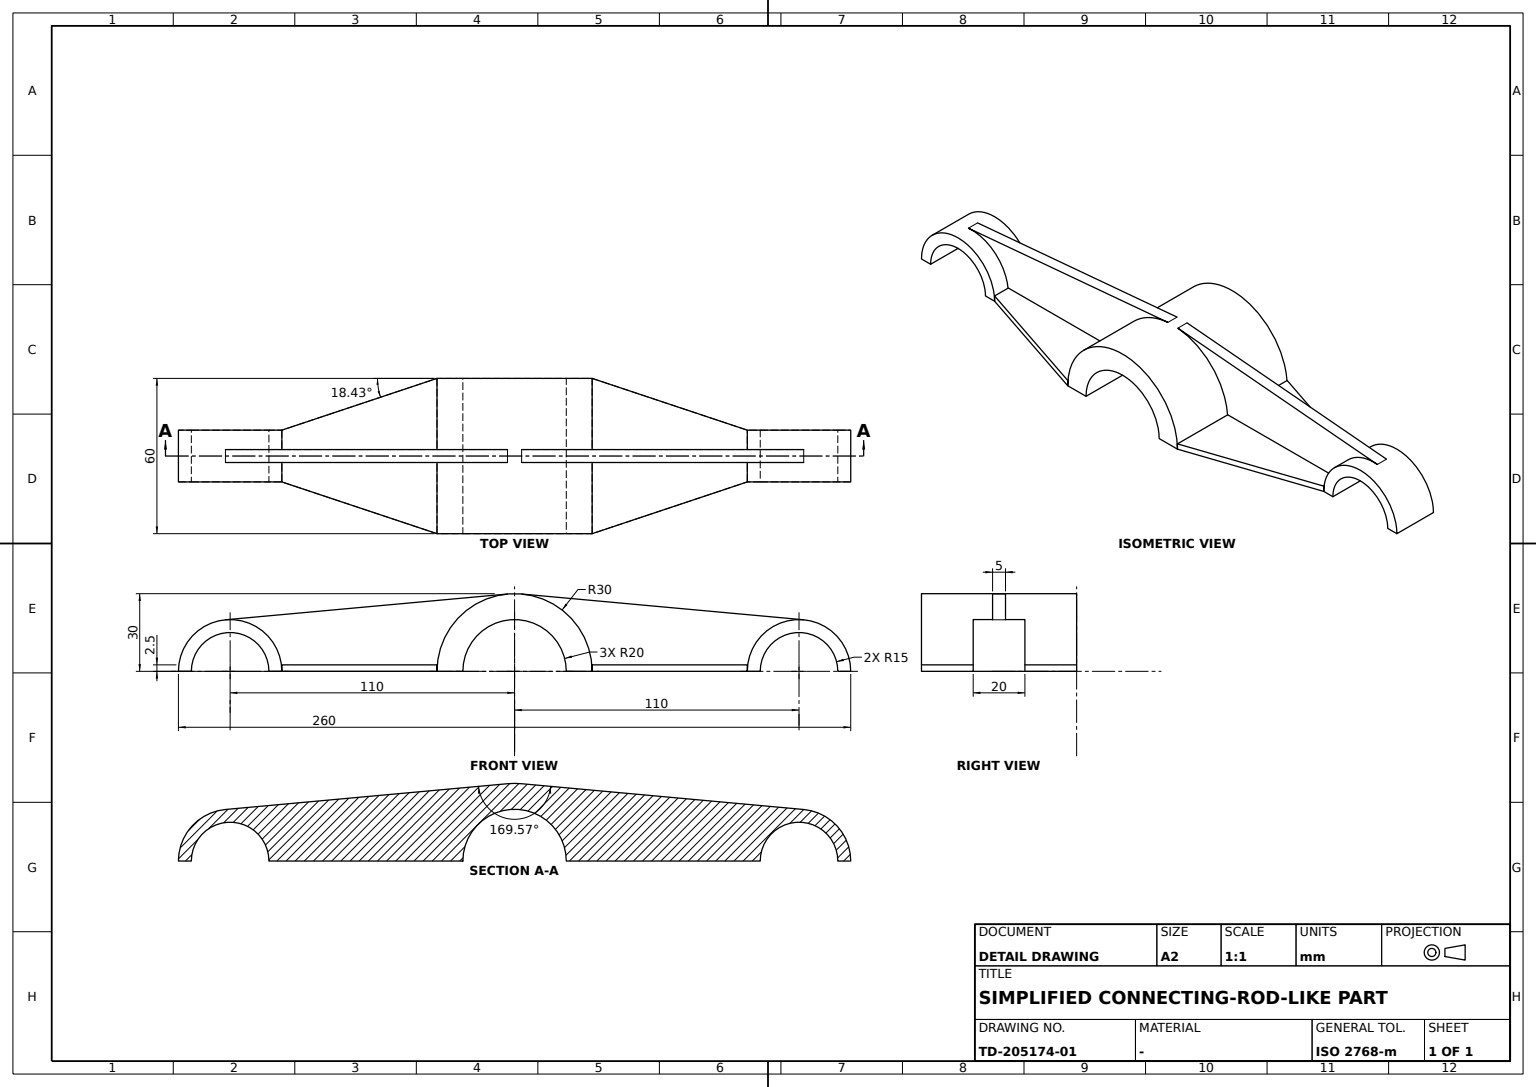
ISO-10303-21;
HEADER;
FILE_DESCRIPTION((''),'2;1');
FILE_NAME('','',(''),(''),'','','');
FILE_SCHEMA(('AUTOMOTIVE_DESIGN'));
ENDSEC;
DATA;
#1=APPLICATION_CONTEXT('');
#2=PRODUCT_CONTEXT('',#1,'mechanical');
#3=PRODUCT('','','',(#2));
#4=PRODUCT_DEFINITION_FORMATION('','',#3);
#5=PRODUCT_DEFINITION_CONTEXT('',#1,'design');
#6=PRODUCT_DEFINITION('','',#4,#5);
#7=PRODUCT_DEFINITION_SHAPE('','',#6);
#8=(LENGTH_UNIT()NAMED_UNIT(*)SI_UNIT(.MILLI.,.METRE.));
#9=(NAMED_UNIT(*)PLANE_ANGLE_UNIT()SI_UNIT($,.RADIAN.));
#10=(NAMED_UNIT(*)SI_UNIT($,.STERADIAN.)SOLID_ANGLE_UNIT());
#11=UNCERTAINTY_MEASURE_WITH_UNIT(LENGTH_MEASURE(0.005),#8,'distance_accuracy_value','');
#12=(GEOMETRIC_REPRESENTATION_CONTEXT(3)GLOBAL_UNCERTAINTY_ASSIGNED_CONTEXT((#11))GLOBAL_UNIT_ASSIGNED_CONTEXT((#8,#9,#10))REPRESENTATION_CONTEXT('',''));
#13=CARTESIAN_POINT('',(20.,-30.,0.));
#14=VERTEX_POINT('',#13);
#15=CARTESIAN_POINT('',(20.,30.,0.));
#16=VERTEX_POINT('',#15);
#17=DIRECTION('',(0.,1.,0.));
#18=VECTOR('',#17,1000.);
#19=LINE('',#13,#18);
#20=EDGE_CURVE('',#14,#16,#19,.T.);
#21=ORIENTED_EDGE('',*,*,#20,.T.);
#22=CARTESIAN_POINT('',(30.,30.,0.));
#23=VERTEX_POINT('',#22);
#24=CARTESIAN_POINT('',(0.,30.,0.));
#25=DIRECTION('',(-1.,0.,0.));
#26=VECTOR('',#25,1000.);
#27=LINE('',#24,#26);
#28=EDGE_CURVE('',#23,#16,#27,.T.);
#29=ORIENTED_EDGE('',*,*,#28,.F.);
#30=CARTESIAN_POINT('',(90.,10.,0.));
#31=VERTEX_POINT('',#30);
#32=DIRECTION('',(0.948683298,-0.316227766,0.));
#33=VECTOR('',#32,1000.);
#34=LINE('',#22,#33);
#35=EDGE_CURVE('',#23,#31,#34,.T.);
#36=ORIENTED_EDGE('',*,*,#35,.T.);
#37=CARTESIAN_POINT('',(95.,10.,0.));
#38=VERTEX_POINT('',#37);
#39=CARTESIAN_POINT('',(30.,10.,0.));
#40=DIRECTION('',(1.,0.,0.));
#41=VECTOR('',#40,1000.);
#42=LINE('',#39,#41);
#43=EDGE_CURVE('',#31,#38,#42,.T.);
#44=ORIENTED_EDGE('',*,*,#43,.T.);
#45=CARTESIAN_POINT('',(95.,-10.,0.));
#46=VERTEX_POINT('',#45);
#47=LINE('',#45,#18);
#48=EDGE_CURVE('',#46,#38,#47,.T.);
#49=ORIENTED_EDGE('',*,*,#48,.F.);
#50=CARTESIAN_POINT('',(90.,-10.,0.));
#51=VERTEX_POINT('',#50);
#52=CARTESIAN_POINT('',(30.,-10.,0.));
#53=LINE('',#52,#41);
#54=EDGE_CURVE('',#51,#46,#53,.T.);
#55=ORIENTED_EDGE('',*,*,#54,.F.);
#56=CARTESIAN_POINT('',(30.,-30.,0.));
#57=VERTEX_POINT('',#56);
#58=DIRECTION('',(0.948683298,0.316227766,0.));
#59=VECTOR('',#58,1000.);
#60=LINE('',#56,#59);
#61=EDGE_CURVE('',#57,#51,#60,.T.);
#62=ORIENTED_EDGE('',*,*,#61,.F.);
#63=CARTESIAN_POINT('',(0.,-30.,0.));
#64=LINE('',#63,#26);
#65=EDGE_CURVE('',#57,#14,#64,.T.);
#66=ORIENTED_EDGE('',*,*,#65,.T.);
#67=EDGE_LOOP('',(#21,#29,#36,#44,#49,#55,#62,#66));
#68=FACE_BOUND('',#67,.T.);
#69=CARTESIAN_POINT('',(30.,0.,0.));
#70=DIRECTION('',(0.,0.,-1.));
#71=AXIS2_PLACEMENT_3D('',#69,#70,#25);
#72=PLANE('',#71);
#73=ADVANCED_FACE('',(#68),#72,.T.);
#74=ORIENTED_EDGE('',*,*,#20,.F.);
#75=CARTESIAN_POINT('',(-20.,-30.,0.));
#76=VERTEX_POINT('',#75);
#77=DIRECTION('',(0.,0.,1.));
#78=AXIS2_PLACEMENT_3D('',#63,#17,#77);
#79=CIRCLE('',#78,20.);
#80=EDGE_CURVE('',#76,#14,#79,.T.);
#81=ORIENTED_EDGE('',*,*,#80,.F.);
#82=CARTESIAN_POINT('',(-20.,30.,0.));
#83=VERTEX_POINT('',#82);
#84=LINE('',#75,#18);
#85=EDGE_CURVE('',#76,#83,#84,.T.);
#86=ORIENTED_EDGE('',*,*,#85,.T.);
#87=AXIS2_PLACEMENT_3D('',#24,#17,#77);
#88=CIRCLE('',#87,20.);
#89=EDGE_CURVE('',#83,#16,#88,.T.);
#90=ORIENTED_EDGE('',*,*,#89,.T.);
#91=EDGE_LOOP('',(#74,#81,#86,#90));
#92=FACE_BOUND('',#91,.T.);
#93=CARTESIAN_POINT('',(0.,0.,0.));
#94=AXIS2_PLACEMENT_3D('',#93,#17,#25);
#95=CYLINDRICAL_SURFACE('',#94,20.);
#96=ADVANCED_FACE('',(#92),#95,.F.);
#97=CARTESIAN_POINT('',(-2.727273,2.5,29.875776));
#98=VERTEX_POINT('',#97);
#99=CARTESIAN_POINT('',(-111.818182,2.5,19.917184));
#100=VERTEX_POINT('',#99);
#101=DIRECTION('',(-0.995859195,0.,-0.090909091));
#102=VECTOR('',#101,1000.);
#103=LINE('',#97,#102);
#104=EDGE_CURVE('',#98,#100,#103,.T.);
#105=ORIENTED_EDGE('',*,*,#104,.T.);
#106=CARTESIAN_POINT('',(-111.818182,-2.5,19.917184));
#107=VERTEX_POINT('',#106);
#108=CARTESIAN_POINT('',(-111.818182,0.,19.917184));
#109=LINE('',#108,#18);
#110=EDGE_CURVE('',#107,#100,#109,.T.);
#111=ORIENTED_EDGE('',*,*,#110,.F.);
#112=CARTESIAN_POINT('',(-2.727273,-2.5,29.875776));
#113=VERTEX_POINT('',#112);
#114=LINE('',#112,#102);
#115=EDGE_CURVE('',#113,#107,#114,.T.);
#116=ORIENTED_EDGE('',*,*,#115,.F.);
#117=CARTESIAN_POINT('',(-2.727273,0.,29.875776));
#118=LINE('',#117,#18);
#119=EDGE_CURVE('',#113,#98,#118,.T.);
#120=ORIENTED_EDGE('',*,*,#119,.T.);
#121=EDGE_LOOP('',(#105,#111,#116,#120));
#122=FACE_BOUND('',#121,.T.);
#123=DIRECTION('',(0.090909091,0.,-0.995859195));
#124=AXIS2_PLACEMENT_3D('',#117,#123,#101);
#125=PLANE('',#124);
#126=ADVANCED_FACE('',(#122),#125,.F.);
#127=CARTESIAN_POINT('',(90.,2.5,0.));
#128=VERTEX_POINT('',#127);
#129=CARTESIAN_POINT('',(90.,0.,0.));
#130=LINE('',#129,#18);
#131=EDGE_CURVE('',#128,#31,#130,.T.);
#132=ORIENTED_EDGE('',*,*,#131,.T.);
#133=CARTESIAN_POINT('',(90.,10.,2.5));
#134=VERTEX_POINT('',#133);
#135=VECTOR('',#77,1000.);
#136=LINE('',#30,#135);
#137=EDGE_CURVE('',#31,#134,#136,.T.);
#138=ORIENTED_EDGE('',*,*,#137,.T.);
#139=CARTESIAN_POINT('',(90.,2.5,2.5));
#140=VERTEX_POINT('',#139);
#141=CARTESIAN_POINT('',(90.,-10.,2.5));
#142=LINE('',#141,#18);
#143=EDGE_CURVE('',#140,#134,#142,.T.);
#144=ORIENTED_EDGE('',*,*,#143,.F.);
#145=LINE('',#127,#135);
#146=EDGE_CURVE('',#128,#140,#145,.T.);
#147=ORIENTED_EDGE('',*,*,#146,.F.);
#148=EDGE_LOOP('',(#132,#138,#144,#147));
#149=FACE_BOUND('',#148,.T.);
#150=AXIS2_PLACEMENT_3D('',#50,#40,#17);
#151=PLANE('',#150);
#152=ADVANCED_FACE('',(#149),#151,.T.);
#153=CARTESIAN_POINT('',(111.818182,2.5,19.917184));
#154=VERTEX_POINT('',#153);
#155=CARTESIAN_POINT('',(110.,2.5,0.));
#156=AXIS2_PLACEMENT_3D('',#155,#17,#77);
#157=CIRCLE('',#156,20.);
#158=EDGE_CURVE('',#128,#154,#157,.T.);
#159=ORIENTED_EDGE('',*,*,#158,.F.);
#160=ORIENTED_EDGE('',*,*,#146,.T.);
#161=CARTESIAN_POINT('',(30.,2.5,2.5));
#162=VERTEX_POINT('',#161);
#163=CARTESIAN_POINT('',(0.,2.5,2.5));
#164=LINE('',#163,#41);
#165=EDGE_CURVE('',#162,#140,#164,.T.);
#166=ORIENTED_EDGE('',*,*,#165,.F.);
#167=CARTESIAN_POINT('',(30.,2.5,0.));
#168=VERTEX_POINT('',#167);
#169=LINE('',#167,#135);
#170=EDGE_CURVE('',#168,#162,#169,.T.);
#171=ORIENTED_EDGE('',*,*,#170,.F.);
#172=CARTESIAN_POINT('',(2.727273,2.5,29.875776));
#173=VERTEX_POINT('',#172);
#174=CARTESIAN_POINT('',(0.,2.5,0.));
#175=AXIS2_PLACEMENT_3D('',#174,#17,#77);
#176=CIRCLE('',#175,30.);
#177=EDGE_CURVE('',#173,#168,#176,.T.);
#178=ORIENTED_EDGE('',*,*,#177,.F.);
#179=DIRECTION('',(0.995859195,0.,-0.090909091));
#180=VECTOR('',#179,1000.);
#181=LINE('',#172,#180);
#182=EDGE_CURVE('',#173,#154,#181,.T.);
#183=ORIENTED_EDGE('',*,*,#182,.T.);
#184=EDGE_LOOP('',(#159,#160,#166,#171,#178,#183));
#185=FACE_BOUND('',#184,.T.);
#186=AXIS2_PLACEMENT_3D('',#174,#17,#25);
#187=PLANE('',#186);
#188=ADVANCED_FACE('',(#185),#187,.T.);
#189=CARTESIAN_POINT('',(-90.,-10.,0.));
#190=VERTEX_POINT('',#189);
#191=CARTESIAN_POINT('',(-90.,-10.,2.5));
#192=VERTEX_POINT('',#191);
#193=LINE('',#189,#135);
#194=EDGE_CURVE('',#190,#192,#193,.T.);
#195=ORIENTED_EDGE('',*,*,#194,.F.);
#196=CARTESIAN_POINT('',(-30.,-30.,0.));
#197=VERTEX_POINT('',#196);
#198=LINE('',#189,#33);
#199=EDGE_CURVE('',#190,#197,#198,.T.);
#200=ORIENTED_EDGE('',*,*,#199,.T.);
#201=CARTESIAN_POINT('',(-30.,-30.,2.5));
#202=VERTEX_POINT('',#201);
#203=LINE('',#196,#135);
#204=EDGE_CURVE('',#197,#202,#203,.T.);
#205=ORIENTED_EDGE('',*,*,#204,.T.);
#206=LINE('',#191,#33);
#207=EDGE_CURVE('',#192,#202,#206,.T.);
#208=ORIENTED_EDGE('',*,*,#207,.F.);
#209=EDGE_LOOP('',(#195,#200,#205,#208));
#210=FACE_BOUND('',#209,.T.);
#211=DIRECTION('',(-0.316227766,-0.948683298,0.));
#212=AXIS2_PLACEMENT_3D('',#189,#211,#32);
#213=PLANE('',#212);
#214=ADVANCED_FACE('',(#210),#213,.T.);
#215=ORIENTED_EDGE('',*,*,#43,.F.);
#216=CARTESIAN_POINT('',(130.,10.,0.));
#217=VERTEX_POINT('',#216);
#218=CARTESIAN_POINT('',(110.,10.,0.));
#219=AXIS2_PLACEMENT_3D('',#218,#17,#77);
#220=CIRCLE('',#219,20.);
#221=EDGE_CURVE('',#31,#217,#220,.T.);
#222=ORIENTED_EDGE('',*,*,#221,.T.);
#223=CARTESIAN_POINT('',(125.,10.,0.));
#224=VERTEX_POINT('',#223);
#225=EDGE_CURVE('',#224,#217,#42,.T.);
#226=ORIENTED_EDGE('',*,*,#225,.F.);
#227=CIRCLE('',#219,15.);
#228=EDGE_CURVE('',#38,#224,#227,.T.);
#229=ORIENTED_EDGE('',*,*,#228,.F.);
#230=EDGE_LOOP('',(#215,#222,#226,#229));
#231=FACE_BOUND('',#230,.T.);
#232=CARTESIAN_POINT('',(0.,10.,0.));
#233=AXIS2_PLACEMENT_3D('',#232,#17,#25);
#234=PLANE('',#233);
#235=ADVANCED_FACE('',(#231),#234,.T.);
#236=ORIENTED_EDGE('',*,*,#104,.F.);
#237=CARTESIAN_POINT('',(-30.,2.5,0.));
#238=VERTEX_POINT('',#237);
#239=EDGE_CURVE('',#238,#98,#176,.T.);
#240=ORIENTED_EDGE('',*,*,#239,.F.);
#241=CARTESIAN_POINT('',(-30.,2.5,2.5));
#242=VERTEX_POINT('',#241);
#243=LINE('',#237,#135);
#244=EDGE_CURVE('',#238,#242,#243,.T.);
#245=ORIENTED_EDGE('',*,*,#244,.T.);
#246=CARTESIAN_POINT('',(-90.,2.5,2.5));
#247=VERTEX_POINT('',#246);
#248=EDGE_CURVE('',#247,#242,#164,.T.);
#249=ORIENTED_EDGE('',*,*,#248,.F.);
#250=CARTESIAN_POINT('',(-90.,2.5,0.));
#251=VERTEX_POINT('',#250);
#252=LINE('',#250,#135);
#253=EDGE_CURVE('',#251,#247,#252,.T.);
#254=ORIENTED_EDGE('',*,*,#253,.F.);
#255=CARTESIAN_POINT('',(-110.,2.5,0.));
#256=AXIS2_PLACEMENT_3D('',#255,#17,#77);
#257=CIRCLE('',#256,20.);
#258=EDGE_CURVE('',#100,#251,#257,.T.);
#259=ORIENTED_EDGE('',*,*,#258,.F.);
#260=EDGE_LOOP('',(#236,#240,#245,#249,#254,#259));
#261=FACE_BOUND('',#260,.T.);
#262=ADVANCED_FACE('',(#261),#187,.T.);
#263=CARTESIAN_POINT('',(-90.,10.,0.));
#264=VERTEX_POINT('',#263);
#265=CARTESIAN_POINT('',(-90.,0.,0.));
#266=LINE('',#265,#18);
#267=EDGE_CURVE('',#251,#264,#266,.T.);
#268=ORIENTED_EDGE('',*,*,#267,.T.);
#269=CARTESIAN_POINT('',(-130.,10.,0.));
#270=VERTEX_POINT('',#269);
#271=CARTESIAN_POINT('',(-110.,10.,0.));
#272=AXIS2_PLACEMENT_3D('',#271,#17,#77);
#273=CIRCLE('',#272,20.);
#274=EDGE_CURVE('',#270,#264,#273,.T.);
#275=ORIENTED_EDGE('',*,*,#274,.F.);
#276=CARTESIAN_POINT('',(-130.,-10.,0.));
#277=VERTEX_POINT('',#276);
#278=LINE('',#276,#18);
#279=EDGE_CURVE('',#277,#270,#278,.T.);
#280=ORIENTED_EDGE('',*,*,#279,.F.);
#281=CARTESIAN_POINT('',(-110.,-10.,0.));
#282=AXIS2_PLACEMENT_3D('',#281,#17,#77);
#283=CIRCLE('',#282,20.);
#284=EDGE_CURVE('',#277,#190,#283,.T.);
#285=ORIENTED_EDGE('',*,*,#284,.T.);
#286=CARTESIAN_POINT('',(-90.,-2.5,0.));
#287=VERTEX_POINT('',#286);
#288=EDGE_CURVE('',#190,#287,#266,.T.);
#289=ORIENTED_EDGE('',*,*,#288,.T.);
#290=CARTESIAN_POINT('',(-110.,-2.5,0.));
#291=AXIS2_PLACEMENT_3D('',#290,#17,#77);
#292=CIRCLE('',#291,20.);
#293=EDGE_CURVE('',#107,#287,#292,.T.);
#294=ORIENTED_EDGE('',*,*,#293,.F.);
#295=ORIENTED_EDGE('',*,*,#110,.T.);
#296=ORIENTED_EDGE('',*,*,#258,.T.);
#297=EDGE_LOOP('',(#268,#275,#280,#285,#289,#294,#295,#296));
#298=FACE_BOUND('',#297,.T.);
#299=CARTESIAN_POINT('',(-110.,0.,0.));
#300=AXIS2_PLACEMENT_3D('',#299,#17,#25);
#301=CYLINDRICAL_SURFACE('',#300,20.);
#302=ADVANCED_FACE('',(#298),#301,.T.);
#303=CARTESIAN_POINT('',(-90.,-2.5,2.5));
#304=VERTEX_POINT('',#303);
#305=LINE('',#191,#18);
#306=EDGE_CURVE('',#192,#304,#305,.T.);
#307=ORIENTED_EDGE('',*,*,#306,.T.);
#308=LINE('',#286,#135);
#309=EDGE_CURVE('',#287,#304,#308,.T.);
#310=ORIENTED_EDGE('',*,*,#309,.F.);
#311=ORIENTED_EDGE('',*,*,#288,.F.);
#312=ORIENTED_EDGE('',*,*,#194,.T.);
#313=EDGE_LOOP('',(#307,#310,#311,#312));
#314=FACE_BOUND('',#313,.T.);
#315=AXIS2_PLACEMENT_3D('',#189,#40,#17);
#316=PLANE('',#315);
#317=ADVANCED_FACE('',(#314),#316,.F.);
#318=CARTESIAN_POINT('',(30.,-2.5,0.));
#319=VERTEX_POINT('',#318);
#320=LINE('',#69,#18);
#321=EDGE_CURVE('',#57,#319,#320,.T.);
#322=ORIENTED_EDGE('',*,*,#321,.T.);
#323=CARTESIAN_POINT('',(2.727273,-2.5,29.875776));
#324=VERTEX_POINT('',#323);
#325=CARTESIAN_POINT('',(0.,-2.5,0.));
#326=AXIS2_PLACEMENT_3D('',#325,#17,#77);
#327=CIRCLE('',#326,30.);
#328=EDGE_CURVE('',#324,#319,#327,.T.);
#329=ORIENTED_EDGE('',*,*,#328,.F.);
#330=CARTESIAN_POINT('',(2.727273,0.,29.875776));
#331=LINE('',#330,#18);
#332=EDGE_CURVE('',#324,#173,#331,.T.);
#333=ORIENTED_EDGE('',*,*,#332,.T.);
#334=ORIENTED_EDGE('',*,*,#177,.T.);
#335=EDGE_CURVE('',#168,#23,#320,.T.);
#336=ORIENTED_EDGE('',*,*,#335,.T.);
#337=CARTESIAN_POINT('',(-30.,30.,0.));
#338=VERTEX_POINT('',#337);
#339=CIRCLE('',#87,30.);
#340=EDGE_CURVE('',#338,#23,#339,.T.);
#341=ORIENTED_EDGE('',*,*,#340,.F.);
#342=CARTESIAN_POINT('',(-30.,0.,0.));
#343=LINE('',#342,#18);
#344=EDGE_CURVE('',#238,#338,#343,.T.);
#345=ORIENTED_EDGE('',*,*,#344,.F.);
#346=ORIENTED_EDGE('',*,*,#239,.T.);
#347=ORIENTED_EDGE('',*,*,#119,.F.);
#348=CARTESIAN_POINT('',(-30.,-2.5,0.));
#349=VERTEX_POINT('',#348);
#350=EDGE_CURVE('',#349,#113,#327,.T.);
#351=ORIENTED_EDGE('',*,*,#350,.F.);
#352=EDGE_CURVE('',#197,#349,#343,.T.);
#353=ORIENTED_EDGE('',*,*,#352,.F.);
#354=CIRCLE('',#78,30.);
#355=EDGE_CURVE('',#197,#57,#354,.T.);
#356=ORIENTED_EDGE('',*,*,#355,.T.);
#357=EDGE_LOOP('',(#322,#329,#333,#334,#336,#341,#345,#346,#347,#351,#353,#356));
#358=FACE_BOUND('',#357,.T.);
#359=CYLINDRICAL_SURFACE('',#94,30.);
#360=ADVANCED_FACE('',(#358),#359,.T.);
#361=ORIENTED_EDGE('',*,*,#65,.F.);
#362=ORIENTED_EDGE('',*,*,#355,.F.);
#363=EDGE_CURVE('',#76,#197,#64,.T.);
#364=ORIENTED_EDGE('',*,*,#363,.F.);
#365=ORIENTED_EDGE('',*,*,#80,.T.);
#366=EDGE_LOOP('',(#361,#362,#364,#365));
#367=FACE_BOUND('',#366,.T.);
#368=AXIS2_PLACEMENT_3D('',#63,#17,#25);
#369=PLANE('',#368);
#370=ADVANCED_FACE('',(#367),#369,.F.);
#371=CARTESIAN_POINT('',(-30.,30.,2.5));
#372=VERTEX_POINT('',#371);
#373=LINE('',#201,#18);
#374=EDGE_CURVE('',#242,#372,#373,.T.);
#375=ORIENTED_EDGE('',*,*,#374,.F.);
#376=ORIENTED_EDGE('',*,*,#244,.F.);
#377=ORIENTED_EDGE('',*,*,#344,.T.);
#378=LINE('',#337,#135);
#379=EDGE_CURVE('',#338,#372,#378,.T.);
#380=ORIENTED_EDGE('',*,*,#379,.T.);
#381=EDGE_LOOP('',(#375,#376,#377,#380));
#382=FACE_BOUND('',#381,.T.);
#383=AXIS2_PLACEMENT_3D('',#196,#40,#17);
#384=PLANE('',#383);
#385=ADVANCED_FACE('',(#382),#384,.T.);
#386=CARTESIAN_POINT('',(30.,-30.,2.5));
#387=VERTEX_POINT('',#386);
#388=LINE('',#56,#135);
#389=EDGE_CURVE('',#57,#387,#388,.T.);
#390=ORIENTED_EDGE('',*,*,#389,.F.);
#391=ORIENTED_EDGE('',*,*,#61,.T.);
#392=VERTEX_POINT('',#141);
#393=LINE('',#50,#135);
#394=EDGE_CURVE('',#51,#392,#393,.T.);
#395=ORIENTED_EDGE('',*,*,#394,.T.);
#396=LINE('',#386,#59);
#397=EDGE_CURVE('',#387,#392,#396,.T.);
#398=ORIENTED_EDGE('',*,*,#397,.F.);
#399=EDGE_LOOP('',(#390,#391,#395,#398));
#400=FACE_BOUND('',#399,.T.);
#401=DIRECTION('',(0.316227766,-0.948683298,0.));
#402=AXIS2_PLACEMENT_3D('',#56,#401,#58);
#403=PLANE('',#402);
#404=ADVANCED_FACE('',(#400),#403,.T.);
#405=CARTESIAN_POINT('',(-90.,10.,2.5));
#406=VERTEX_POINT('',#405);
#407=EDGE_CURVE('',#247,#406,#305,.T.);
#408=ORIENTED_EDGE('',*,*,#407,.F.);
#409=ORIENTED_EDGE('',*,*,#248,.T.);
#410=ORIENTED_EDGE('',*,*,#374,.T.);
#411=DIRECTION('',(-0.948683298,-0.316227766,0.));
#412=VECTOR('',#411,1000.);
#413=LINE('',#371,#412);
#414=EDGE_CURVE('',#372,#406,#413,.T.);
#415=ORIENTED_EDGE('',*,*,#414,.T.);
#416=EDGE_LOOP('',(#408,#409,#410,#415));
#417=FACE_BOUND('',#416,.T.);
#418=CARTESIAN_POINT('',(0.,0.,2.5));
#419=AXIS2_PLACEMENT_3D('',#418,#70,#40);
#420=PLANE('',#419);
#421=ADVANCED_FACE('',(#417),#420,.F.);
#422=CARTESIAN_POINT('',(90.,-2.5,0.));
#423=VERTEX_POINT('',#422);
#424=EDGE_CURVE('',#51,#423,#130,.T.);
#425=ORIENTED_EDGE('',*,*,#424,.T.);
#426=CARTESIAN_POINT('',(90.,-2.5,2.5));
#427=VERTEX_POINT('',#426);
#428=LINE('',#422,#135);
#429=EDGE_CURVE('',#423,#427,#428,.T.);
#430=ORIENTED_EDGE('',*,*,#429,.T.);
#431=EDGE_CURVE('',#392,#427,#142,.T.);
#432=ORIENTED_EDGE('',*,*,#431,.F.);
#433=ORIENTED_EDGE('',*,*,#394,.F.);
#434=EDGE_LOOP('',(#425,#430,#432,#433));
#435=FACE_BOUND('',#434,.T.);
#436=ADVANCED_FACE('',(#435),#151,.T.);
#437=ORIENTED_EDGE('',*,*,#431,.T.);
#438=CARTESIAN_POINT('',(30.,-2.5,2.5));
#439=VERTEX_POINT('',#438);
#440=CARTESIAN_POINT('',(0.,-2.5,2.5));
#441=LINE('',#440,#41);
#442=EDGE_CURVE('',#439,#427,#441,.T.);
#443=ORIENTED_EDGE('',*,*,#442,.F.);
#444=LINE('',#386,#18);
#445=EDGE_CURVE('',#387,#439,#444,.T.);
#446=ORIENTED_EDGE('',*,*,#445,.F.);
#447=ORIENTED_EDGE('',*,*,#397,.T.);
#448=EDGE_LOOP('',(#437,#443,#446,#447));
#449=FACE_BOUND('',#448,.T.);
#450=ADVANCED_FACE('',(#449),#420,.F.);
#451=CARTESIAN_POINT('',(125.,-10.,0.));
#452=VERTEX_POINT('',#451);
#453=CARTESIAN_POINT('',(110.,-10.,0.));
#454=AXIS2_PLACEMENT_3D('',#453,#17,#77);
#455=CIRCLE('',#454,15.);
#456=EDGE_CURVE('',#46,#452,#455,.T.);
#457=ORIENTED_EDGE('',*,*,#456,.T.);
#458=CARTESIAN_POINT('',(130.,-10.,0.));
#459=VERTEX_POINT('',#458);
#460=EDGE_CURVE('',#452,#459,#53,.T.);
#461=ORIENTED_EDGE('',*,*,#460,.T.);
#462=CIRCLE('',#454,20.);
#463=EDGE_CURVE('',#51,#459,#462,.T.);
#464=ORIENTED_EDGE('',*,*,#463,.F.);
#465=ORIENTED_EDGE('',*,*,#54,.T.);
#466=EDGE_LOOP('',(#457,#461,#464,#465));
#467=FACE_BOUND('',#466,.T.);
#468=CARTESIAN_POINT('',(0.,-10.,0.));
#469=AXIS2_PLACEMENT_3D('',#468,#17,#25);
#470=PLANE('',#469);
#471=ADVANCED_FACE('',(#467),#470,.F.);
#472=ORIENTED_EDGE('',*,*,#352,.T.);
#473=CARTESIAN_POINT('',(-30.,-2.5,2.5));
#474=VERTEX_POINT('',#473);
#475=LINE('',#348,#135);
#476=EDGE_CURVE('',#349,#474,#475,.T.);
#477=ORIENTED_EDGE('',*,*,#476,.T.);
#478=EDGE_CURVE('',#202,#474,#373,.T.);
#479=ORIENTED_EDGE('',*,*,#478,.F.);
#480=ORIENTED_EDGE('',*,*,#204,.F.);
#481=EDGE_LOOP('',(#472,#477,#479,#480));
#482=FACE_BOUND('',#481,.T.);
#483=ADVANCED_FACE('',(#482),#384,.T.);
#484=ORIENTED_EDGE('',*,*,#89,.F.);
#485=EDGE_CURVE('',#83,#338,#27,.T.);
#486=ORIENTED_EDGE('',*,*,#485,.T.);
#487=ORIENTED_EDGE('',*,*,#340,.T.);
#488=ORIENTED_EDGE('',*,*,#28,.T.);
#489=EDGE_LOOP('',(#484,#486,#487,#488));
#490=FACE_BOUND('',#489,.T.);
#491=AXIS2_PLACEMENT_3D('',#24,#17,#25);
#492=PLANE('',#491);
#493=ADVANCED_FACE('',(#490),#492,.T.);
#494=LINE('',#263,#135);
#495=EDGE_CURVE('',#264,#406,#494,.T.);
#496=ORIENTED_EDGE('',*,*,#495,.F.);
#497=ORIENTED_EDGE('',*,*,#267,.F.);
#498=ORIENTED_EDGE('',*,*,#253,.T.);
#499=ORIENTED_EDGE('',*,*,#407,.T.);
#500=EDGE_LOOP('',(#496,#497,#498,#499));
#501=FACE_BOUND('',#500,.T.);
#502=ADVANCED_FACE('',(#501),#316,.F.);
#503=ORIENTED_EDGE('',*,*,#460,.F.);
#504=LINE('',#451,#18);
#505=EDGE_CURVE('',#452,#224,#504,.T.);
#506=ORIENTED_EDGE('',*,*,#505,.T.);
#507=ORIENTED_EDGE('',*,*,#225,.T.);
#508=LINE('',#458,#18);
#509=EDGE_CURVE('',#459,#217,#508,.T.);
#510=ORIENTED_EDGE('',*,*,#509,.F.);
#511=EDGE_LOOP('',(#503,#506,#507,#510));
#512=FACE_BOUND('',#511,.T.);
#513=ADVANCED_FACE('',(#512),#72,.T.);
#514=CARTESIAN_POINT('',(-95.,-10.,0.));
#515=VERTEX_POINT('',#514);
#516=CARTESIAN_POINT('',(-95.,10.,0.));
#517=VERTEX_POINT('',#516);
#518=LINE('',#514,#18);
#519=EDGE_CURVE('',#515,#517,#518,.T.);
#520=ORIENTED_EDGE('',*,*,#519,.F.);
#521=CARTESIAN_POINT('',(-125.,-10.,0.));
#522=VERTEX_POINT('',#521);
#523=CIRCLE('',#282,15.);
#524=EDGE_CURVE('',#522,#515,#523,.T.);
#525=ORIENTED_EDGE('',*,*,#524,.F.);
#526=CARTESIAN_POINT('',(-125.,10.,0.));
#527=VERTEX_POINT('',#526);
#528=LINE('',#521,#18);
#529=EDGE_CURVE('',#522,#527,#528,.T.);
#530=ORIENTED_EDGE('',*,*,#529,.T.);
#531=CIRCLE('',#272,15.);
#532=EDGE_CURVE('',#527,#517,#531,.T.);
#533=ORIENTED_EDGE('',*,*,#532,.T.);
#534=EDGE_LOOP('',(#520,#525,#530,#533));
#535=FACE_BOUND('',#534,.T.);
#536=CYLINDRICAL_SURFACE('',#300,15.);
#537=ADVANCED_FACE('',(#535),#536,.F.);
#538=CARTESIAN_POINT('',(30.,30.,2.5));
#539=VERTEX_POINT('',#538);
#540=EDGE_CURVE('',#162,#539,#444,.T.);
#541=ORIENTED_EDGE('',*,*,#540,.T.);
#542=LINE('',#22,#135);
#543=EDGE_CURVE('',#23,#539,#542,.T.);
#544=ORIENTED_EDGE('',*,*,#543,.F.);
#545=ORIENTED_EDGE('',*,*,#335,.F.);
#546=ORIENTED_EDGE('',*,*,#170,.T.);
#547=EDGE_LOOP('',(#541,#544,#545,#546));
#548=FACE_BOUND('',#547,.T.);
#549=AXIS2_PLACEMENT_3D('',#56,#40,#17);
#550=PLANE('',#549);
#551=ADVANCED_FACE('',(#548),#550,.F.);
#552=ORIENTED_EDGE('',*,*,#543,.T.);
#553=LINE('',#538,#33);
#554=EDGE_CURVE('',#539,#134,#553,.T.);
#555=ORIENTED_EDGE('',*,*,#554,.T.);
#556=ORIENTED_EDGE('',*,*,#137,.F.);
#557=ORIENTED_EDGE('',*,*,#35,.F.);
#558=EDGE_LOOP('',(#552,#555,#556,#557));
#559=FACE_BOUND('',#558,.T.);
#560=AXIS2_PLACEMENT_3D('',#22,#211,#32);
#561=PLANE('',#560);
#562=ADVANCED_FACE('',(#559),#561,.F.);
#563=CARTESIAN_POINT('',(111.818182,-2.5,19.917184));
#564=VERTEX_POINT('',#563);
#565=CARTESIAN_POINT('',(110.,-2.5,0.));
#566=AXIS2_PLACEMENT_3D('',#565,#17,#77);
#567=CIRCLE('',#566,20.);
#568=EDGE_CURVE('',#423,#564,#567,.T.);
#569=ORIENTED_EDGE('',*,*,#568,.F.);
#570=ORIENTED_EDGE('',*,*,#424,.F.);
#571=ORIENTED_EDGE('',*,*,#463,.T.);
#572=ORIENTED_EDGE('',*,*,#509,.T.);
#573=ORIENTED_EDGE('',*,*,#221,.F.);
#574=ORIENTED_EDGE('',*,*,#131,.F.);
#575=ORIENTED_EDGE('',*,*,#158,.T.);
#576=CARTESIAN_POINT('',(111.818182,0.,19.917184));
#577=LINE('',#576,#18);
#578=EDGE_CURVE('',#564,#154,#577,.T.);
#579=ORIENTED_EDGE('',*,*,#578,.F.);
#580=EDGE_LOOP('',(#569,#570,#571,#572,#573,#574,#575,#579));
#581=FACE_BOUND('',#580,.T.);
#582=CARTESIAN_POINT('',(110.,0.,0.));
#583=AXIS2_PLACEMENT_3D('',#582,#17,#25);
#584=CYLINDRICAL_SURFACE('',#583,20.);
#585=ADVANCED_FACE('',(#581),#584,.T.);
#586=EDGE_CURVE('',#517,#264,#42,.T.);
#587=ORIENTED_EDGE('',*,*,#586,.F.);
#588=ORIENTED_EDGE('',*,*,#532,.F.);
#589=EDGE_CURVE('',#270,#527,#42,.T.);
#590=ORIENTED_EDGE('',*,*,#589,.F.);
#591=ORIENTED_EDGE('',*,*,#274,.T.);
#592=EDGE_LOOP('',(#587,#588,#590,#591));
#593=FACE_BOUND('',#592,.T.);
#594=ADVANCED_FACE('',(#593),#234,.T.);
#595=ORIENTED_EDGE('',*,*,#456,.F.);
#596=ORIENTED_EDGE('',*,*,#48,.T.);
#597=ORIENTED_EDGE('',*,*,#228,.T.);
#598=ORIENTED_EDGE('',*,*,#505,.F.);
#599=EDGE_LOOP('',(#595,#596,#597,#598));
#600=FACE_BOUND('',#599,.T.);
#601=CYLINDRICAL_SURFACE('',#583,15.);
#602=ADVANCED_FACE('',(#600),#601,.F.);
#603=ORIENTED_EDGE('',*,*,#389,.T.);
#604=ORIENTED_EDGE('',*,*,#445,.T.);
#605=LINE('',#318,#135);
#606=EDGE_CURVE('',#319,#439,#605,.T.);
#607=ORIENTED_EDGE('',*,*,#606,.F.);
#608=ORIENTED_EDGE('',*,*,#321,.F.);
#609=EDGE_LOOP('',(#603,#604,#607,#608));
#610=FACE_BOUND('',#609,.T.);
#611=ADVANCED_FACE('',(#610),#550,.F.);
#612=ORIENTED_EDGE('',*,*,#442,.T.);
#613=ORIENTED_EDGE('',*,*,#429,.F.);
#614=ORIENTED_EDGE('',*,*,#568,.T.);
#615=LINE('',#323,#180);
#616=EDGE_CURVE('',#324,#564,#615,.T.);
#617=ORIENTED_EDGE('',*,*,#616,.F.);
#618=ORIENTED_EDGE('',*,*,#328,.T.);
#619=ORIENTED_EDGE('',*,*,#606,.T.);
#620=EDGE_LOOP('',(#612,#613,#614,#617,#618,#619));
#621=FACE_BOUND('',#620,.T.);
#622=AXIS2_PLACEMENT_3D('',#325,#17,#25);
#623=PLANE('',#622);
#624=ADVANCED_FACE('',(#621),#623,.F.);
#625=ORIENTED_EDGE('',*,*,#85,.F.);
#626=ORIENTED_EDGE('',*,*,#363,.T.);
#627=ORIENTED_EDGE('',*,*,#199,.F.);
#628=EDGE_CURVE('',#515,#190,#53,.T.);
#629=ORIENTED_EDGE('',*,*,#628,.F.);
#630=ORIENTED_EDGE('',*,*,#519,.T.);
#631=ORIENTED_EDGE('',*,*,#586,.T.);
#632=LINE('',#337,#412);
#633=EDGE_CURVE('',#338,#264,#632,.T.);
#634=ORIENTED_EDGE('',*,*,#633,.F.);
#635=ORIENTED_EDGE('',*,*,#485,.F.);
#636=EDGE_LOOP('',(#625,#626,#627,#629,#630,#631,#634,#635));
#637=FACE_BOUND('',#636,.T.);
#638=ADVANCED_FACE('',(#637),#72,.T.);
#639=ORIENTED_EDGE('',*,*,#616,.T.);
#640=ORIENTED_EDGE('',*,*,#578,.T.);
#641=ORIENTED_EDGE('',*,*,#182,.F.);
#642=ORIENTED_EDGE('',*,*,#332,.F.);
#643=EDGE_LOOP('',(#639,#640,#641,#642));
#644=FACE_BOUND('',#643,.T.);
#645=DIRECTION('',(0.090909091,0.,0.995859195));
#646=AXIS2_PLACEMENT_3D('',#330,#645,#179);
#647=PLANE('',#646);
#648=ADVANCED_FACE('',(#644),#647,.T.);
#649=ORIENTED_EDGE('',*,*,#165,.T.);
#650=ORIENTED_EDGE('',*,*,#143,.T.);
#651=ORIENTED_EDGE('',*,*,#554,.F.);
#652=ORIENTED_EDGE('',*,*,#540,.F.);
#653=EDGE_LOOP('',(#649,#650,#651,#652));
#654=FACE_BOUND('',#653,.T.);
#655=ADVANCED_FACE('',(#654),#420,.F.);
#656=ORIENTED_EDGE('',*,*,#379,.F.);
#657=ORIENTED_EDGE('',*,*,#633,.T.);
#658=ORIENTED_EDGE('',*,*,#495,.T.);
#659=ORIENTED_EDGE('',*,*,#414,.F.);
#660=EDGE_LOOP('',(#656,#657,#658,#659));
#661=FACE_BOUND('',#660,.T.);
#662=DIRECTION('',(-0.316227766,0.948683298,0.));
#663=AXIS2_PLACEMENT_3D('',#337,#662,#411);
#664=PLANE('',#663);
#665=ADVANCED_FACE('',(#661),#664,.T.);
#666=EDGE_CURVE('',#304,#474,#441,.T.);
#667=ORIENTED_EDGE('',*,*,#666,.T.);
#668=ORIENTED_EDGE('',*,*,#476,.F.);
#669=ORIENTED_EDGE('',*,*,#350,.T.);
#670=ORIENTED_EDGE('',*,*,#115,.T.);
#671=ORIENTED_EDGE('',*,*,#293,.T.);
#672=ORIENTED_EDGE('',*,*,#309,.T.);
#673=EDGE_LOOP('',(#667,#668,#669,#670,#671,#672));
#674=FACE_BOUND('',#673,.T.);
#675=ADVANCED_FACE('',(#674),#623,.F.);
#676=ORIENTED_EDGE('',*,*,#529,.F.);
#677=EDGE_CURVE('',#277,#522,#53,.T.);
#678=ORIENTED_EDGE('',*,*,#677,.F.);
#679=ORIENTED_EDGE('',*,*,#279,.T.);
#680=ORIENTED_EDGE('',*,*,#589,.T.);
#681=EDGE_LOOP('',(#676,#678,#679,#680));
#682=FACE_BOUND('',#681,.T.);
#683=ADVANCED_FACE('',(#682),#72,.T.);
#684=ORIENTED_EDGE('',*,*,#628,.T.);
#685=ORIENTED_EDGE('',*,*,#284,.F.);
#686=ORIENTED_EDGE('',*,*,#677,.T.);
#687=ORIENTED_EDGE('',*,*,#524,.T.);
#688=EDGE_LOOP('',(#684,#685,#686,#687));
#689=FACE_BOUND('',#688,.T.);
#690=ADVANCED_FACE('',(#689),#470,.F.);
#691=ORIENTED_EDGE('',*,*,#666,.F.);
#692=ORIENTED_EDGE('',*,*,#306,.F.);
#693=ORIENTED_EDGE('',*,*,#207,.T.);
#694=ORIENTED_EDGE('',*,*,#478,.T.);
#695=EDGE_LOOP('',(#691,#692,#693,#694));
#696=FACE_BOUND('',#695,.T.);
#697=ADVANCED_FACE('',(#696),#420,.F.);
#698=CLOSED_SHELL('',(#73,#96,#126,#152,#188,#214,#235,#262,#302,#317,#360,#370,#385,#404,#421,#436,#450,#471,#483,#493,#502,#513,#537,#551,#562,#585,#594,#602,#611,#624,#638,#648,#655,#665,#675,#683,#690,#697));
#699=MANIFOLD_SOLID_BREP('',#698);
#700=ADVANCED_BREP_SHAPE_REPRESENTATION('',(#699),#12);
#701=SHAPE_DEFINITION_REPRESENTATION(#7,#700);
ENDSEC;
END-ISO-10303-21;
